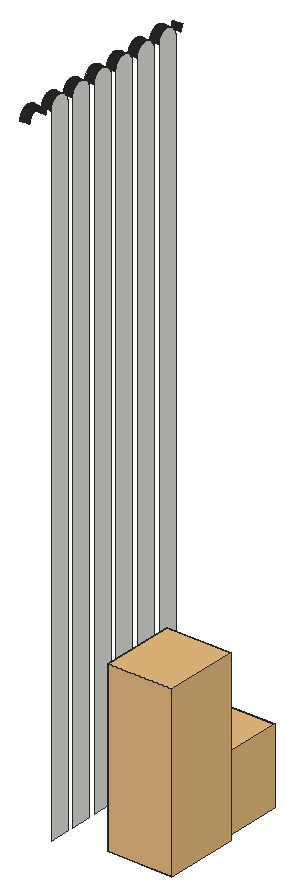
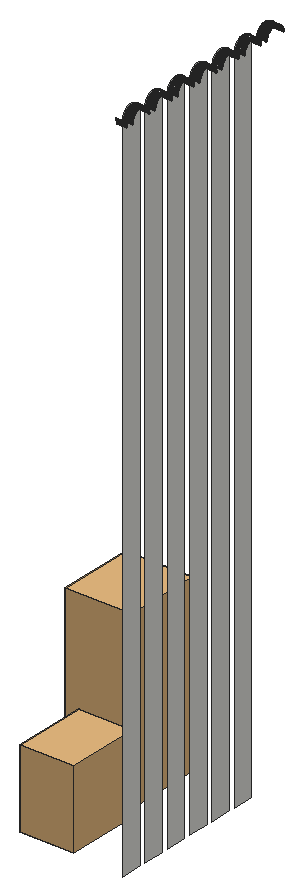
# SketchUp Ruby script. Lengths in inches.
U = 1.inch
M = Sketchup.active_model
def pt(a) = Geom::Point3d.new(a.map { |v| v * U })
def face(e, loops, mat)
  f = e.add_face(loops[0].map { |a| pt(a) })
  loops[1..].each { |l| e.add_face(l.map { |a| pt(a) }).erase! }
  f.material = f.back_material = mat if mat
  f
end
# faces: each face lists its corners as indices into pts; further lists are holes
def faces(e, pts, list, mat = nil) = list.each { |f| face(e, (f[0].is_a?(Array) ? f : [f]).map { |l| l.map { |i| pts[i] } }, mat) }
# xy, xz, yz: faces in a plane at the given z, y or x. An outline is a flat list of corners, or four numbers for a rectangle; further outlines are holes
def ring(l) = l.size == 4 ? [[l[0], l[1]], [l[2], l[1]], [l[2], l[3]], [l[0], l[3]]] : l.each_slice(2).to_a
def flat(e, list, mat, &to3) = list.each { |f| face(e, (f[0].is_a?(Array) ? f : [f]).map { |l| ring(l).map { |u, v| to3.(u, v) } }, mat) }
def xy(e, z, list, mat = nil) = flat(e, list, mat) { |x, y| [x, y, z] }
def xz(e, y, list, mat = nil) = flat(e, list, mat) { |x, z| [x, y, z] }
def yz(e, x, list, mat = nil) = flat(e, list, mat) { |y, z| [x, y, z] }
def lines(e, pts, list) = list.each { |a, b| e.add_line(pt(pts[a]), pt(pts[b])) }
# prism: a flat outline (further loops are holes) pulled along v
def prism(e, loops, v, mat = nil)
  f = face(e, loops, mat); d = Geom::Vector3d.new(v.map { |x| x * U })
  f.pushpull(f.normal.samedirection?(d) ? d.length : -d.length)
end
def box(e, o, s, mat = nil) = prism(e, [[o, [o[0] + s[0], o[1], o[2]], [o[0] + s[0], o[1] + s[1], o[2]], [o[0], o[1] + s[1], o[2]]]], [0, 0, s[2]], mat)
def at(x, y, z, deg = 0) = Geom::Transformation.translation(pt([x, y, z])) * Geom::Transformation.rotation(ORIGIN, Z_AXIS, deg.degrees)
def axes(o, x, y, z) = Geom::Transformation.new([*x, 0, *y, 0, *z, 0, *pt(o).to_a, 1])
def part(name) = M.definitions.add(name)
# library, detail: a bought-in or finely detailed component or shape, given as its bounding box
def library(name, o, s) = part(name).tap { |d| box(d.entities, o, s) }
def detail(e, o, s) = box(e.add_group.entities, o, s)
def put(e, d, t, mat = nil) = e.add_instance(d, t).tap { |i| i.material = mat if mat }
def group(e, t, mat = nil) = e.add_group.tap { |g| g.transformation = t; g.material = mat if mat }.entities
root = M.entities
c1 = library("skpA613",[-33.11,-37.89,-86.79],[66.22,75.78,173.58])
c2 = library("Decoração+Banheiro",[28.69,-29.77,58.91],[5.39,6.58,5.91])
xy(root,108,[[9,16.217,10,16.326],[9,19.005,10,19.114],[9,21.792,10,21.901],[9,24.58,10,24.689],[9,27.367,10,27.476],
  [9,30.155,10,30.264],[9,32.942,10,33.051]])
yz(root,9,[[16.217,108,16.326,108,16.272,108.001],[19.005,108,19.114,108,19.059,108.001],[21.792,108,21.901,108,21.847,108.001],[24.58,108,24.689,108,24.634,108.001],[27.367,108,27.476,108,27.422,108.001],
  [30.155,108,30.264,108,30.209,108.001],[32.942,108,33.051,108,32.997,108.001]])
yz(root,10,[[18.018,39.466,20.1,39.466,20.1,106.961,20.099,107.015,20.094,107.069,20.087,107.123,20.077,107.177,20.065,107.23,20.049,107.282,20.031,107.334,20.01,107.384,19.987,107.433,19.961,107.481,19.932,107.528,19.901,107.572,19.868,107.616,19.833,107.657,19.795,107.697,19.756,107.734,19.714,107.769,19.671,107.803,19.626,107.834,19.58,107.862,19.532,107.888,19.483,107.911,19.432,107.932,19.381,107.95,19.329,107.966,19.276,107.979,19.222,107.989,19.168,107.996,19.114,108,19.005,108,18.95,107.996,18.896,107.989,18.843,107.979,18.79,107.966,18.738,107.95,18.686,107.932,18.636,107.911,18.587,107.888,18.539,107.862,18.492,107.834,18.448,107.803,18.404,107.769,18.363,107.734,18.323,107.697,18.286,107.657,18.25,107.616,18.217,107.572,18.186,107.528,18.158,107.481,18.132,107.433,18.108,107.384,18.088,107.334,18.069,107.282,18.054,107.23,18.041,107.177,18.031,107.123,18.024,107.069,18.02,107.015,18.018,106.961],[20.806,39.466,22.887,39.466,22.887,106.961,22.886,107.015,22.882,107.069,22.875,107.123,22.865,107.177,22.852,107.23,22.837,107.282,22.818,107.334,22.798,107.384,22.774,107.433,22.748,107.481,22.72,107.528,22.689,107.572,22.656,107.616,22.62,107.657,22.583,107.697,22.543,107.734,22.502,107.769,22.458,107.803,22.414,107.834,22.367,107.862,22.319,107.888,22.27,107.911,22.22,107.932,22.168,107.95,22.116,107.966,22.063,107.979,22.01,107.989,21.956,107.996,21.901,108,21.792,108,21.738,107.996,21.684,107.989,21.63,107.979,21.577,107.966,21.525,107.95,21.474,107.932,21.423,107.911,21.374,107.888,21.326,107.862,21.28,107.834,21.235,107.803,21.192,107.769,21.15,107.734,21.111,107.697,21.073,107.657,21.038,107.616,21.005,107.572,20.974,107.528,20.945,107.481,20.919,107.433,20.896,107.384,20.875,107.334,20.857,107.282,20.841,107.23,20.829,107.177,20.819,107.123,20.812,107.069,20.807,107.015,20.806,106.961],[23.593,39.466,25.675,39.466,25.675,106.961,25.674,107.015,25.669,107.069,25.662,107.123,25.652,107.177,25.64,107.23,25.624,107.282,25.606,107.334,25.585,107.384,25.562,107.433,25.536,107.481,25.507,107.528,25.476,107.572,25.443,107.616,25.408,107.657,25.37,107.697,25.331,107.734,25.289,107.769,25.246,107.803,25.201,107.834,25.155,107.862,25.107,107.888,25.058,107.911,25.007,107.932,24.956,107.95,24.904,107.966,24.851,107.979,24.797,107.989,24.743,107.996,24.689,108,24.58,108,24.525,107.996,24.471,107.989,24.418,107.979,24.365,107.966,24.3125,107.95,24.261,107.932,24.211,107.911,24.162,107.888,24.114,107.862,24.067,107.834,24.023,107.803,23.979,107.769,23.938,107.734,23.898,107.697,23.861,107.657,23.825,107.616,23.792,107.572,23.761,107.528,23.733,107.481,23.707,107.433,23.683,107.384,23.663,107.334,23.644,107.282,23.629,107.23,23.616,107.177,23.606,107.123,23.599,107.069,23.595,107.015,23.593,106.961],[26.381,39.466,28.462,39.466,28.462,106.961,28.461,107.015,28.457,107.069,28.45,107.123,28.44,107.177,28.427,107.23,28.412,107.282,28.393,107.334,28.373,107.384,28.349,107.433,28.323,107.481,28.295,107.528,28.264,107.572,28.231,107.616,28.195,107.657,28.158,107.697,28.118,107.734,28.077,107.769,28.033,107.803,27.989,107.834,27.942,107.862,27.894,107.888,27.845,107.911,27.795,107.932,27.743,107.95,27.691,107.966,27.638,107.979,27.585,107.989,27.531,107.996,27.476,108,27.367,108,27.313,107.996,27.259,107.989,27.205,107.979,27.152,107.966,27.1,107.95,27.049,107.932,26.998,107.911,26.949,107.888,26.901,107.862,26.855,107.834,26.81,107.803,26.767,107.769,26.725,107.734,26.686,107.697,26.648,107.657,26.613,107.616,26.58,107.572,26.549,107.528,26.52,107.481,26.494,107.433,26.471,107.384,26.45,107.334,26.432,107.282,26.416,107.23,26.404,107.177,26.394,107.123,26.387,107.069,26.382,107.015,26.381,106.961],[29.168,39.466,31.25,39.466,31.25,106.961,31.249,107.015,31.244,107.069,31.237,107.123,31.227,107.177,31.215,107.23,31.199,107.282,31.181,107.334,31.16,107.384,31.137,107.433,31.111,107.481,31.082,107.528,31.051,107.572,31.018,107.616,30.983,107.657,30.945,107.697,30.906,107.734,30.864,107.769,30.821,107.803,30.776,107.834,30.73,107.862,30.682,107.888,30.633,107.911,30.582,107.932,30.531,107.95,30.479,107.966,30.426,107.979,30.372,107.989,30.318,107.996,30.264,108,30.155,108,30.1,107.996,30.046,107.989,29.993,107.979,29.94,107.966,29.888,107.95,29.836,107.932,29.786,107.911,29.737,107.888,29.689,107.862,29.642,107.834,29.598,107.803,29.554,107.769,29.513,107.734,29.473,107.697,29.436,107.657,29.4,107.616,29.367,107.572,29.336,107.528,29.308,107.481,29.282,107.433,29.258,107.384,29.238,107.334,29.219,107.282,29.204,107.23,29.191,107.177,29.181,107.123,29.174,107.069,29.17,107.015,29.168,106.961],
  [31.956,39.466,34.037,39.466,34.037,106.961,34.036,107.015,34.032,107.069,34.025,107.123,34.015,107.177,34.002,107.23,33.987,107.282,33.968,107.334,33.948,107.384,33.924,107.433,33.898,107.481,33.87,107.528,33.839,107.572,33.806,107.616,33.77,107.657,33.733,107.697,33.693,107.734,33.652,107.769,33.608,107.803,33.564,107.834,33.517,107.862,33.469,107.888,33.42,107.911,33.37,107.932,33.318,107.95,33.266,107.966,33.213,107.979,33.16,107.989,33.106,107.996,33.051,108,32.942,108,32.888,107.996,32.834,107.989,32.78,107.979,32.727,107.966,32.675,107.95,32.624,107.932,32.573,107.911,32.524,107.888,32.476,107.862,32.43,107.834,32.385,107.803,32.342,107.769,32.3,107.734,32.261,107.697,32.223,107.657,32.188,107.616,32.155,107.572,32.124,107.528,32.095,107.481,32.069,107.433,32.046,107.384,32.025,107.334,32.007,107.282,31.991,107.23,31.979,107.177,31.969,107.123,31.962,107.069,31.957,107.015,31.956,106.961]])
p = [[9,15.232,107.015],[9,15.231,106.961],[10,15.231,106.961],[10,15.232,107.015],[9,15.237,107.069],[10,15.237,107.069],
  [9,17.311,107.015],[9,17.307,107.069],[10,17.307,107.069],[10,17.311,107.015],[9,17.3125,106.961],[10,17.3125,106.961],
  [9,18.02,107.015],[9,18.018,106.961],[10,18.018,106.961],[10,18.02,107.015],[9,18.024,107.069],[10,18.024,107.069],
  [9,20.099,107.015],[9,20.094,107.069],[10,20.094,107.069],[10,20.099,107.015],[9,20.1,106.961],[10,20.1,106.961],
  [9,20.807,107.015],[9,20.806,106.961],[10,20.806,106.961],[10,20.807,107.015],[9,20.812,107.069],[10,20.812,107.069],
  [9,22.886,107.015],[9,22.882,107.069],[10,22.882,107.069],[10,22.886,107.015],[9,22.887,106.961],[10,22.887,106.961],
  [9,23.595,107.015],[9,23.593,106.961],[10,23.593,106.961],[10,23.595,107.015],[9,23.599,107.069],[10,23.599,107.069],
  [9,25.674,107.015],[9,25.669,107.069],[10,25.669,107.069],[10,25.674,107.015],[9,25.675,106.961],[10,25.675,106.961],
  [9,26.382,107.015],[9,26.381,106.961],[10,26.381,106.961],[10,26.382,107.015],[9,26.387,107.069],[10,26.387,107.069],
  [9,28.461,107.015],[9,28.457,107.069],[10,28.457,107.069],[10,28.461,107.015],[9,28.462,106.961],[10,28.462,106.961],
  [9,29.17,107.015],[9,29.168,106.961],[10,29.168,106.961],[10,29.17,107.015],[9,29.174,107.069],[10,29.174,107.069],
  [9,31.249,107.015],[9,31.244,107.069],[10,31.244,107.069],[10,31.249,107.015],[9,31.25,106.961],[10,31.25,106.961],
  [9,31.957,107.015],[9,31.956,106.961],[10,31.956,106.961],[10,31.957,107.015],[9,31.962,107.069],[10,31.962,107.069],
  [9,34.036,107.015],[9,34.032,107.069],[10,34.032,107.069],[10,34.036,107.015],[9,34.037,106.961],[10,34.037,106.961],
  [9,34.745,107.015],[9,34.743,106.961],[10,34.743,106.961],[10,34.745,107.015],[9,34.749,107.069],[10,34.749,107.069],
  [9,15.244,107.123],[10,15.244,107.123],[9,15.254,107.177],[10,15.254,107.177],[9,17.3,107.123],[9,17.29,107.177],
  [10,17.29,107.177],[10,17.3,107.123],[9,18.031,107.123],[10,18.031,107.123],[9,18.041,107.177],[10,18.041,107.177],
  [9,20.087,107.123],[9,20.077,107.177],[10,20.077,107.177],[10,20.087,107.123],[9,20.819,107.123],[10,20.819,107.123],
  [9,20.829,107.177],[10,20.829,107.177],[9,22.875,107.123],[9,22.865,107.177],[10,22.865,107.177],[10,22.875,107.123],
  [9,23.606,107.123],[10,23.606,107.123],[9,23.616,107.177],[10,23.616,107.177],[9,25.662,107.123],[9,25.652,107.177],
  [10,25.652,107.177],[10,25.662,107.123],[9,26.394,107.123],[10,26.394,107.123],[9,26.404,107.177],[10,26.404,107.177],
  [9,28.45,107.123],[9,28.44,107.177],[10,28.44,107.177],[10,28.45,107.123],[9,29.181,107.123],[10,29.181,107.123],
  [9,29.191,107.177],[10,29.191,107.177],[9,31.237,107.123],[9,31.227,107.177],[10,31.227,107.177],[10,31.237,107.123],
  [9,31.969,107.123],[10,31.969,107.123],[9,31.979,107.177],[10,31.979,107.177],[9,34.025,107.123],[9,34.015,107.177],
  [10,34.015,107.177],[10,34.025,107.123],[9,34.756,107.123],[10,34.756,107.123],[9,34.766,107.177],[10,34.766,107.177],
  [9,15.266,107.23],[10,15.266,107.23],[9,15.282,107.282],[10,15.282,107.282],[9,17.277,107.23],[9,17.262,107.282],
  [10,17.262,107.282],[10,17.277,107.23],[9,18.054,107.23],[10,18.054,107.23],[9,18.069,107.282],[10,18.069,107.282],
  [9,20.065,107.23],[9,20.049,107.282],[10,20.049,107.282],[10,20.065,107.23],[9,20.841,107.23],[10,20.841,107.23],
  [9,20.857,107.282],[10,20.857,107.282],[9,22.852,107.23],[9,22.837,107.282],[10,22.837,107.282],[10,22.852,107.23],
  [9,23.629,107.23],[10,23.629,107.23],[9,23.644,107.282],[10,23.644,107.282],[9,25.64,107.23],[9,25.624,107.282],
  [10,25.624,107.282],[10,25.64,107.23],[9,26.416,107.23],[10,26.416,107.23],[9,26.432,107.282],[10,26.432,107.282],
  [9,28.427,107.23],[9,28.412,107.282],[10,28.412,107.282],[10,28.427,107.23],[9,29.204,107.23],[10,29.204,107.23],
  [9,29.219,107.282],[10,29.219,107.282],[9,31.215,107.23],[9,31.199,107.282],[10,31.199,107.282],[10,31.215,107.23],
  [9,31.991,107.23],[10,31.991,107.23],[9,32.007,107.282],[10,32.007,107.282],[9,34.002,107.23],[9,33.987,107.282],
  [10,33.987,107.282],[10,34.002,107.23],[9,34.779,107.23],[10,34.779,107.23],[9,34.794,107.282],[10,34.794,107.282],
  [9,15.3,107.334],[10,15.3,107.334],[9,15.321,107.384],[10,15.321,107.384],[9,17.243,107.334],[9,17.223,107.384],
  [10,17.223,107.384],[10,17.243,107.334],[9,18.088,107.334],[10,18.088,107.334],[9,18.108,107.384],[10,18.108,107.384],
  [9,20.031,107.334],[9,20.01,107.384],[10,20.01,107.384],[10,20.031,107.334],[9,20.875,107.334],[10,20.875,107.334],
  [9,20.896,107.384],[10,20.896,107.384],[9,22.818,107.334],[9,22.798,107.384],[10,22.798,107.384],[10,22.818,107.334],
  [9,23.663,107.334],[10,23.663,107.334],[9,23.683,107.384],[10,23.683,107.384],[9,25.606,107.334],[9,25.585,107.384],
  [10,25.585,107.384],[10,25.606,107.334],[9,26.45,107.334],[10,26.45,107.334],[9,26.471,107.384],[10,26.471,107.384],
  [9,28.393,107.334],[9,28.373,107.384],[10,28.373,107.384],[10,28.393,107.334],[9,29.238,107.334],[10,29.238,107.334],
  [9,29.258,107.384],[10,29.258,107.384],[9,31.181,107.334],[9,31.16,107.384],[10,31.16,107.384],[10,31.181,107.334],
  [9,32.025,107.334],[10,32.025,107.334],[9,32.046,107.384],[10,32.046,107.384],[9,33.968,107.334],[9,33.948,107.384],
  [10,33.948,107.384],[10,33.968,107.334],[9,34.8125,107.334],[10,34.8125,107.334],[9,34.833,107.384],[10,34.833,107.384],
  [9,15.344,107.433],[10,15.344,107.433],[9,15.37,107.481],[10,15.37,107.481],[9,17.199,107.433],[9,17.173,107.481],
  [10,17.173,107.481],[10,17.199,107.433],[9,18.132,107.433],[10,18.132,107.433],[9,18.158,107.481],[10,18.158,107.481],
  [9,19.987,107.433],[9,19.961,107.481],[10,19.961,107.481],[10,19.987,107.433],[9,20.919,107.433],[10,20.919,107.433],
  [9,20.945,107.481],[10,20.945,107.481],[9,22.774,107.433],[9,22.748,107.481],[10,22.748,107.481],[10,22.774,107.433],
  [9,23.707,107.433],[10,23.707,107.433],[9,23.733,107.481],[10,23.733,107.481],[9,25.562,107.433],[9,25.536,107.481],
  [10,25.536,107.481],[10,25.562,107.433],[9,26.494,107.433],[10,26.494,107.433],[9,26.52,107.481],[10,26.52,107.481],
  [9,28.349,107.433],[9,28.323,107.481],[10,28.323,107.481],[10,28.349,107.433],[9,29.282,107.433],[10,29.282,107.433],
  [9,29.308,107.481],[10,29.308,107.481],[9,31.137,107.433],[9,31.111,107.481],[10,31.111,107.481],[10,31.137,107.433],
  [9,32.069,107.433],[10,32.069,107.433],[9,32.095,107.481],[10,32.095,107.481],[9,33.924,107.433],[9,33.898,107.481],
  [10,33.898,107.481],[10,33.924,107.433],[9,34.857,107.433],[10,34.857,107.433],[9,34.883,107.481],[10,34.883,107.481],
  [9,15.399,107.528],[10,15.399,107.528],[9,15.43,107.572],[10,15.43,107.572],[9,17.145,107.528],[9,17.114,107.572],
  [10,17.114,107.572],[10,17.145,107.528],[9,18.186,107.528],[10,18.186,107.528],[9,18.217,107.572],[10,18.217,107.572],
  [9,19.932,107.528],[9,19.901,107.572],[10,19.901,107.572],[10,19.932,107.528],[9,20.974,107.528],[10,20.974,107.528],
  [9,21.005,107.572],[10,21.005,107.572],[9,22.72,107.528],[9,22.689,107.572],[10,22.689,107.572],[10,22.72,107.528],
  [9,23.761,107.528],[10,23.761,107.528],[9,23.792,107.572],[10,23.792,107.572],[9,25.507,107.528],[9,25.476,107.572],
  [10,25.476,107.572],[10,25.507,107.528],[9,26.549,107.528],[10,26.549,107.528],[9,26.58,107.572],[10,26.58,107.572],
  [9,28.295,107.528],[9,28.264,107.572],[10,28.264,107.572],[10,28.295,107.528],[9,29.336,107.528],[10,29.336,107.528],
  [9,29.367,107.572],[10,29.367,107.572],[9,31.082,107.528],[9,31.051,107.572],[10,31.051,107.572],[10,31.082,107.528],
  [9,32.124,107.528],[10,32.124,107.528],[9,32.155,107.572],[10,32.155,107.572],[9,33.87,107.528],[9,33.839,107.572],
  [10,33.839,107.572],[10,33.87,107.528],[9,34.911,107.528],[10,34.911,107.528],[9,34.942,107.572],[10,34.942,107.572],
  [9,15.463,107.616],[10,15.463,107.616],[9,15.498,107.657],[10,15.498,107.657],[9,17.081,107.616],[9,17.045,107.657],
  [10,17.045,107.657],[10,17.081,107.616],[9,18.25,107.616],[10,18.25,107.616],[9,18.286,107.657],[10,18.286,107.657],
  [9,19.868,107.616],[9,19.833,107.657],[10,19.833,107.657],[10,19.868,107.616],[9,21.038,107.616],[10,21.038,107.616],
  [9,21.073,107.657],[10,21.073,107.657],[9,22.656,107.616],[9,22.62,107.657],[10,22.62,107.657],[10,22.656,107.616],
  [9,23.825,107.616],[10,23.825,107.616],[9,23.861,107.657],[10,23.861,107.657],[9,25.443,107.616],[9,25.408,107.657],
  [10,25.408,107.657],[10,25.443,107.616],[9,26.613,107.616],[10,26.613,107.616],[9,26.648,107.657],[10,26.648,107.657],
  [9,28.231,107.616],[9,28.195,107.657],[10,28.195,107.657],[10,28.231,107.616],[9,29.4,107.616],[10,29.4,107.616],
  [9,29.436,107.657],[10,29.436,107.657],[9,31.018,107.616],[9,30.983,107.657],[10,30.983,107.657],[10,31.018,107.616],
  [9,32.188,107.616],[10,32.188,107.616],[9,32.223,107.657],[10,32.223,107.657],[9,33.806,107.616],[9,33.77,107.657],
  [10,33.77,107.657],[10,33.806,107.616],[9,15.536,107.697],[10,15.536,107.697],[9,15.575,107.734],[10,15.575,107.734],
  [9,15.617,107.769],[10,15.617,107.769],[9,16.968,107.734],[9,16.927,107.769],[10,16.927,107.769],[10,16.968,107.734],
  [9,17.008,107.697],[10,17.008,107.697],[9,18.323,107.697],[10,18.323,107.697],[9,18.363,107.734],[10,18.363,107.734],
  [9,18.404,107.769],[10,18.404,107.769],[9,19.756,107.734],[9,19.714,107.769],[10,19.714,107.769],[10,19.756,107.734],
  [9,19.795,107.697],[10,19.795,107.697],[9,21.111,107.697],[10,21.111,107.697],[9,21.15,107.734],[10,21.15,107.734],
  [9,21.192,107.769],[10,21.192,107.769],[9,22.543,107.734],[9,22.502,107.769],[10,22.502,107.769],[10,22.543,107.734],
  [9,22.583,107.697],[10,22.583,107.697],[9,23.898,107.697],[10,23.898,107.697],[9,23.938,107.734],[10,23.938,107.734],
  [9,23.979,107.769],[10,23.979,107.769],[9,25.331,107.734],[9,25.289,107.769],[10,25.289,107.769],[10,25.331,107.734],
  [9,25.37,107.697],[10,25.37,107.697],[9,26.686,107.697],[10,26.686,107.697],[9,26.725,107.734],[10,26.725,107.734],
  [9,26.767,107.769],[10,26.767,107.769],[9,28.118,107.734],[9,28.077,107.769],[10,28.077,107.769],[10,28.118,107.734],
  [9,28.158,107.697],[10,28.158,107.697],[9,29.473,107.697],[10,29.473,107.697],[9,29.513,107.734],[10,29.513,107.734],
  [9,29.554,107.769],[10,29.554,107.769],[9,30.906,107.734],[9,30.864,107.769],[10,30.864,107.769],[10,30.906,107.734],
  [9,30.945,107.697],[10,30.945,107.697],[9,32.261,107.697],[10,32.261,107.697],[9,32.3,107.734],[10,32.3,107.734],
  [9,32.342,107.769],[10,32.342,107.769],[9,33.693,107.734],[9,33.652,107.769],[10,33.652,107.769],[10,33.693,107.734],
  [9,33.733,107.697],[10,33.733,107.697],[9,15.66,107.803],[10,15.66,107.803],[9,15.705,107.834],[10,15.705,107.834],
  [9,15.751,107.862],[10,15.751,107.862],[9,16.839,107.834],[9,16.792,107.862],[10,16.792,107.862],[10,16.839,107.834],
  [9,16.883,107.803],[10,16.883,107.803],[9,18.448,107.803],[10,18.448,107.803],[9,18.492,107.834],[10,18.492,107.834],
  [9,18.539,107.862],[10,18.539,107.862],[9,19.626,107.834],[9,19.58,107.862],[10,19.58,107.862],[10,19.626,107.834],
  [9,19.671,107.803],[10,19.671,107.803],[9,21.235,107.803],[10,21.235,107.803],[9,21.28,107.834],[10,21.28,107.834],
  [9,21.326,107.862],[10,21.326,107.862],[9,22.414,107.834],[9,22.367,107.862],[10,22.367,107.862],[10,22.414,107.834],
  [9,22.458,107.803],[10,22.458,107.803],[9,24.023,107.803],[10,24.023,107.803],[9,24.067,107.834],[10,24.067,107.834],
  [9,24.114,107.862],[10,24.114,107.862],[9,25.201,107.834],[9,25.155,107.862],[10,25.155,107.862],[10,25.201,107.834],
  [9,25.246,107.803],[10,25.246,107.803],[9,26.81,107.803],[10,26.81,107.803],[9,26.855,107.834],[10,26.855,107.834],
  [9,26.901,107.862],[10,26.901,107.862],[9,27.989,107.834],[9,27.942,107.862],[10,27.942,107.862],[10,27.989,107.834],
  [9,28.033,107.803],[10,28.033,107.803],[9,29.598,107.803],[10,29.598,107.803],[9,29.642,107.834],[10,29.642,107.834],
  [9,29.689,107.862],[10,29.689,107.862],[9,30.776,107.834],[9,30.73,107.862],[10,30.73,107.862],[10,30.776,107.834],
  [9,30.821,107.803],[10,30.821,107.803],[9,32.385,107.803],[10,32.385,107.803],[9,32.43,107.834],[10,32.43,107.834],
  [9,32.476,107.862],[10,32.476,107.862],[9,33.564,107.834],[9,33.517,107.862],[10,33.517,107.862],[10,33.564,107.834],
  [9,33.608,107.803],[10,33.608,107.803],[9,15.799,107.888],[10,15.799,107.888],[9,15.848,107.911],[10,15.848,107.911],
  [9,15.899,107.932],[10,15.899,107.932],[9,15.95,107.95],[10,15.95,107.95],[9,16.645,107.932],[9,16.593,107.95],
  [10,16.593,107.95],[10,16.645,107.932],[9,16.695,107.911],[10,16.695,107.911],[9,16.744,107.888],[10,16.744,107.888],
  [9,18.587,107.888],[10,18.587,107.888],[9,18.636,107.911],[10,18.636,107.911],[9,18.686,107.932],[10,18.686,107.932],
  [9,18.738,107.95],[10,18.738,107.95],[9,19.432,107.932],[9,19.381,107.95],[10,19.381,107.95],[10,19.432,107.932],
  [9,19.483,107.911],[10,19.483,107.911],[9,19.532,107.888],[10,19.532,107.888],[9,21.374,107.888],[10,21.374,107.888],
  [9,21.423,107.911],[10,21.423,107.911],[9,21.474,107.932],[10,21.474,107.932],[9,21.525,107.95],[10,21.525,107.95],
  [9,22.22,107.932],[9,22.168,107.95],[10,22.168,107.95],[10,22.22,107.932],[9,22.27,107.911],[10,22.27,107.911],
  [9,22.319,107.888],[10,22.319,107.888],[9,24.162,107.888],[10,24.162,107.888],[9,24.211,107.911],[10,24.211,107.911],
  [9,24.261,107.932],[10,24.261,107.932],[9,24.3125,107.95],[10,24.3125,107.95],[9,25.007,107.932],[9,24.956,107.95],
  [10,24.956,107.95],[10,25.007,107.932],[9,25.058,107.911],[10,25.058,107.911],[9,25.107,107.888],[10,25.107,107.888],
  [9,26.949,107.888],[10,26.949,107.888],[9,26.998,107.911],[10,26.998,107.911],[9,27.049,107.932],[10,27.049,107.932],
  [9,27.1,107.95],[10,27.1,107.95],[9,27.795,107.932],[9,27.743,107.95],[10,27.743,107.95],[10,27.795,107.932],
  [9,27.845,107.911],[10,27.845,107.911],[9,27.894,107.888],[10,27.894,107.888],[9,29.737,107.888],[10,29.737,107.888],
  [9,29.786,107.911],[10,29.786,107.911],[9,29.836,107.932],[10,29.836,107.932],[9,29.888,107.95],[10,29.888,107.95],
  [9,30.582,107.932],[9,30.531,107.95],[10,30.531,107.95],[10,30.582,107.932],[9,30.633,107.911],[10,30.633,107.911],
  [9,30.682,107.888],[10,30.682,107.888],[9,32.524,107.888],[10,32.524,107.888],[9,32.573,107.911],[10,32.573,107.911],
  [9,32.624,107.932],[10,32.624,107.932],[9,32.675,107.95],[10,32.675,107.95],[9,33.37,107.932],[9,33.318,107.95],
  [10,33.318,107.95],[10,33.37,107.932],[9,33.42,107.911],[10,33.42,107.911],[9,33.469,107.888],[10,33.469,107.888],
  [9,16.002,107.966],[10,16.002,107.966],[9,16.055,107.979],[10,16.055,107.979],[9,16.109,107.989],[10,16.109,107.989],
  [9,16.163,107.996],[10,16.163,107.996],[9,16.217,108],[10,16.217,108],[9,16.381,107.996],[9,16.326,108],
  [10,16.326,108],[10,16.381,107.996],[9,16.435,107.989],[10,16.435,107.989],[9,16.488,107.979],[10,16.488,107.979],
  [9,16.541,107.966],[10,16.541,107.966],[9,18.79,107.966],[10,18.79,107.966],[9,18.843,107.979],[10,18.843,107.979],
  [9,18.896,107.989],[10,18.896,107.989],[9,18.95,107.996],[10,18.95,107.996],[9,19.005,108],[10,19.005,108],
  [9,19.168,107.996],[9,19.114,108],[10,19.114,108],[10,19.168,107.996],[9,19.222,107.989],[10,19.222,107.989],
  [9,19.276,107.979],[10,19.276,107.979],[9,19.329,107.966],[10,19.329,107.966],[9,21.577,107.966],[10,21.577,107.966],
  [9,21.63,107.979],[10,21.63,107.979],[9,21.684,107.989],[10,21.684,107.989],[9,21.738,107.996],[10,21.738,107.996],
  [9,21.792,108],[10,21.792,108],[9,21.956,107.996],[9,21.901,108],[10,21.901,108],[10,21.956,107.996],
  [9,22.01,107.989],[10,22.01,107.989],[9,22.063,107.979],[10,22.063,107.979],[9,22.116,107.966],[10,22.116,107.966],
  [9,24.365,107.966],[10,24.365,107.966],[9,24.418,107.979],[10,24.418,107.979],[9,24.471,107.989],[10,24.471,107.989],
  [9,24.525,107.996],[10,24.525,107.996],[9,24.58,108],[10,24.58,108],[9,24.743,107.996],[9,24.689,108],
  [10,24.689,108],[10,24.743,107.996],[9,24.797,107.989],[10,24.797,107.989],[9,24.851,107.979],[10,24.851,107.979],
  [9,24.904,107.966],[10,24.904,107.966],[9,27.152,107.966],[10,27.152,107.966],[9,27.205,107.979],[10,27.205,107.979],
  [9,27.259,107.989],[10,27.259,107.989],[9,27.313,107.996],[10,27.313,107.996],[9,27.367,108],[10,27.367,108],
  [9,27.531,107.996],[9,27.476,108],[10,27.476,108],[10,27.531,107.996],[9,27.585,107.989],[10,27.585,107.989],
  [9,27.638,107.979],[10,27.638,107.979],[9,27.691,107.966],[10,27.691,107.966],[9,29.94,107.966],[10,29.94,107.966],
  [9,29.993,107.979],[10,29.993,107.979],[9,30.046,107.989],[10,30.046,107.989],[9,30.1,107.996],[10,30.1,107.996],
  [9,30.155,108],[10,30.155,108],[9,30.318,107.996],[9,30.264,108],[10,30.264,108],[10,30.318,107.996],
  [9,30.372,107.989],[10,30.372,107.989],[9,30.426,107.979],[10,30.426,107.979],[9,30.479,107.966],[10,30.479,107.966],
  [9,32.727,107.966],[10,32.727,107.966],[9,32.78,107.979],[10,32.78,107.979],[9,32.834,107.989],[10,32.834,107.989],
  [9,32.888,107.996],[10,32.888,107.996],[9,32.942,108],[10,32.942,108],[9,33.106,107.996],[9,33.051,108],
  [10,33.051,108],[10,33.106,107.996],[9,33.16,107.989],[10,33.16,107.989],[9,33.213,107.979],[10,33.213,107.979],
  [9,33.266,107.966],[10,33.266,107.966],[9,18.018,39.466],[8.9375,18.018,39.466]]
faces(root,p,[[0,1,2,3],[4,0,3,5],[6,7,8,9],[10,6,9,11],[12,13,14,15],[16,12,15,17],[18,19,20,21],[22,18,21,23],
  [24,25,26,27],[28,24,27,29],[30,31,32,33],[34,30,33,35],[36,37,38,39],[40,36,39,41],[42,43,44,45],[46,42,45,47],
  [48,49,50,51],[52,48,51,53],[54,55,56,57],[58,54,57,59],[60,61,62,63],[64,60,63,65],[66,67,68,69],[70,66,69,71],
  [72,73,74,75],[76,72,75,77],[78,79,80,81],[82,78,81,83],[84,85,86,87],[88,84,87,89],[90,4,5,91],[92,90,91,93],
  [94,95,96,97],[7,94,97,8],[98,16,17,99],[100,98,99,101],[102,103,104,105],[19,102,105,20],[106,28,29,107],[108,106,107,109],
  [110,111,112,113],[31,110,113,32],[114,40,41,115],[116,114,115,117],[118,119,120,121],[43,118,121,44],[122,52,53,123],[124,122,123,125],
  [126,127,128,129],[55,126,129,56],[130,64,65,131],[132,130,131,133],[134,135,136,137],[67,134,137,68],[138,76,77,139],[140,138,139,141],
  [142,143,144,145],[79,142,145,80],[146,88,89,147],[148,146,147,149],[150,92,93,151],[152,150,151,153],[154,155,156,157],[95,154,157,96],
  [158,100,101,159],[160,158,159,161],[162,163,164,165],[103,162,165,104],[166,108,109,167],[168,166,167,169],[170,171,172,173],[111,170,173,112],
  [174,116,117,175],[176,174,175,177],[178,179,180,181],[119,178,181,120],[182,124,125,183],[184,182,183,185],[186,187,188,189],[127,186,189,128],
  [190,132,133,191],[192,190,191,193],[194,195,196,197],[135,194,197,136],[198,140,141,199],[200,198,199,201],[202,203,204,205],[143,202,205,144],
  [206,148,149,207],[208,206,207,209],[210,152,153,211],[212,210,211,213],[214,215,216,217],[155,214,217,156],[218,160,161,219],[220,218,219,221],
  [222,223,224,225],[163,222,225,164],[226,168,169,227],[228,226,227,229],[230,231,232,233],[171,230,233,172],[234,176,177,235],[236,234,235,237],
  [238,239,240,241],[179,238,241,180],[242,184,185,243],[244,242,243,245],[246,247,248,249],[187,246,249,188],[250,192,193,251],[252,250,251,253],
  [254,255,256,257],[195,254,257,196],[258,200,201,259],[260,258,259,261],[262,263,264,265],[203,262,265,204],[266,208,209,267],[268,266,267,269],
  [270,212,213,271],[272,270,271,273],[274,275,276,277],[215,274,277,216],[278,220,221,279],[280,278,279,281],[282,283,284,285],[223,282,285,224],
  [286,228,229,287],[288,286,287,289],[290,291,292,293],[231,290,293,232],[294,236,237,295],[296,294,295,297],[298,299,300,301],[239,298,301,240],
  [302,244,245,303],[304,302,303,305],[306,307,308,309],[247,306,309,248],[310,252,253,311],[312,310,311,313],[314,315,316,317],[255,314,317,256],
  [318,260,261,319],[320,318,319,321],[322,323,324,325],[263,322,325,264],[326,268,269,327],[328,326,327,329],[330,272,273,331],[332,330,331,333],
  [334,335,336,337],[275,334,337,276],[338,280,281,339],[340,338,339,341],[342,343,344,345],[283,342,345,284],[346,288,289,347],[348,346,347,349],
  [350,351,352,353],[291,350,353,292],[354,296,297,355],[356,354,355,357],[358,359,360,361],[299,358,361,300],[362,304,305,363],[364,362,363,365],
  [366,367,368,369],[307,366,369,308],[370,312,313,371],[372,370,371,373],[374,375,376,377],[315,374,377,316],[378,320,321,379],[380,378,379,381],
  [382,383,384,385],[323,382,385,324],[386,328,329,387],[388,386,387,389],[390,332,333,391],[392,390,391,393],[394,395,396,397],[335,394,397,336],
  [398,340,341,399],[400,398,399,401],[402,403,404,405],[343,402,405,344],[406,348,349,407],[408,406,407,409],[410,411,412,413],[351,410,413,352],
  [414,356,357,415],[416,414,415,417],[418,419,420,421],[359,418,421,360],[422,364,365,423],[424,422,423,425],[426,427,428,429],[367,426,429,368],
  [430,372,373,431],[432,430,431,433],[434,435,436,437],[375,434,437,376],[438,380,381,439],[440,438,439,441],[442,443,444,445],[383,442,445,384],
  [446,392,393,447],[448,446,447,449],[450,448,449,451],[452,453,454,455],[456,452,455,457],[395,456,457,396],[458,400,401,459],[460,458,459,461],
  [462,460,461,463],[464,465,466,467],[468,464,467,469],[403,468,469,404],[470,408,409,471],[472,470,471,473],[474,472,473,475],[476,477,478,479],
  [480,476,479,481],[411,480,481,412],[482,416,417,483],[484,482,483,485],[486,484,485,487],[488,489,490,491],[492,488,491,493],[419,492,493,420],
  [494,424,425,495],[496,494,495,497],[498,496,497,499],[500,501,502,503],[504,500,503,505],[427,504,505,428],[506,432,433,507],[508,506,507,509],
  [510,508,509,511],[512,513,514,515],[516,512,515,517],[435,516,517,436],[518,440,441,519],[520,518,519,521],[522,520,521,523],[524,525,526,527],
  [528,524,527,529],[443,528,529,444],[530,450,451,531],[532,530,531,533],[534,532,533,535],[536,537,538,539],[540,536,539,541],[453,540,541,454],
  [542,462,463,543],[544,542,543,545],[546,544,545,547],[548,549,550,551],[552,548,551,553],[465,552,553,466],[554,474,475,555],[556,554,555,557],
  [558,556,557,559],[560,561,562,563],[564,560,563,565],[477,564,565,478],[566,486,487,567],[568,566,567,569],[570,568,569,571],[572,573,574,575],
  [576,572,575,577],[489,576,577,490],[578,498,499,579],[580,578,579,581],[582,580,581,583],[584,585,586,587],[588,584,587,589],[501,588,589,502],
  [590,510,511,591],[592,590,591,593],[594,592,593,595],[596,597,598,599],[600,596,599,601],[513,600,601,514],[602,522,523,603],[604,602,603,605],
  [606,604,605,607],[608,609,610,611],[612,608,611,613],[525,612,613,526],[614,534,535,615],[616,614,615,617],[618,616,617,619],[620,618,619,621],
  [622,623,624,625],[626,622,625,627],[628,626,627,629],[537,628,629,538],[630,546,547,631],[632,630,631,633],[634,632,633,635],[636,634,635,637],
  [638,639,640,641],[642,638,641,643],[644,642,643,645],[549,644,645,550],[646,558,559,647],[648,646,647,649],[650,648,649,651],[652,650,651,653],
  [654,655,656,657],[658,654,657,659],[660,658,659,661],[561,660,661,562],[662,570,571,663],[664,662,663,665],[666,664,665,667],[668,666,667,669],
  [670,671,672,673],[674,670,673,675],[676,674,675,677],[573,676,677,574],[678,582,583,679],[680,678,679,681],[682,680,681,683],[684,682,683,685],
  [686,687,688,689],[690,686,689,691],[692,690,691,693],[585,692,693,586],[694,594,595,695],[696,694,695,697],[698,696,697,699],[700,698,699,701],
  [702,703,704,705],[706,702,705,707],[708,706,707,709],[597,708,709,598],[710,606,607,711],[712,710,711,713],[714,712,713,715],[716,714,715,717],
  [718,719,720,721],[722,718,721,723],[724,722,723,725],[609,724,725,610],[726,620,621,727],[728,726,727,729],[730,728,729,731],[732,730,731,733],
  [734,732,733,735],[736,737,738,739],[740,736,739,741],[742,740,741,743],[744,742,743,745],[623,744,745,624],[746,636,637,747],[748,746,747,749],
  [750,748,749,751],[752,750,751,753],[754,752,753,755],[756,757,758,759],[760,756,759,761],[762,760,761,763],[764,762,763,765],[639,764,765,640],
  [766,652,653,767],[768,766,767,769],[770,768,769,771],[772,770,771,773],[774,772,773,775],[776,777,778,779],[780,776,779,781],[782,780,781,783],
  [784,782,783,785],[655,784,785,656],[786,668,669,787],[788,786,787,789],[790,788,789,791],[792,790,791,793],[794,792,793,795],[796,797,798,799],
  [800,796,799,801],[802,800,801,803],[804,802,803,805],[671,804,805,672],[806,684,685,807],[808,806,807,809],[810,808,809,811],[812,810,811,813],
  [814,812,813,815],[816,817,818,819],[820,816,819,821],[822,820,821,823],[824,822,823,825],[687,824,825,688],[826,700,701,827],[828,826,827,829],
  [830,828,829,831],[832,830,831,833],[834,832,833,835],[836,837,838,839],[840,836,839,841],[842,840,841,843],[844,842,843,845],[703,844,845,704],
  [846,716,717,847],[848,846,847,849],[850,848,849,851],[852,850,851,853],[854,852,853,855],[856,857,858,859],[860,856,859,861],[862,860,861,863],
  [864,862,863,865],[719,864,865,720]])
lines(root,p,[[866,867]])
put(root,c1,axes([18.73,22.36,48.83],[0.1,0,0],[0,0.1,0],[0,0,0.1]))
put(root,c2,axes([-13.4,59.45,-37.71],[1,0,0],[0,1.12,0],[0,0,1.31]))
